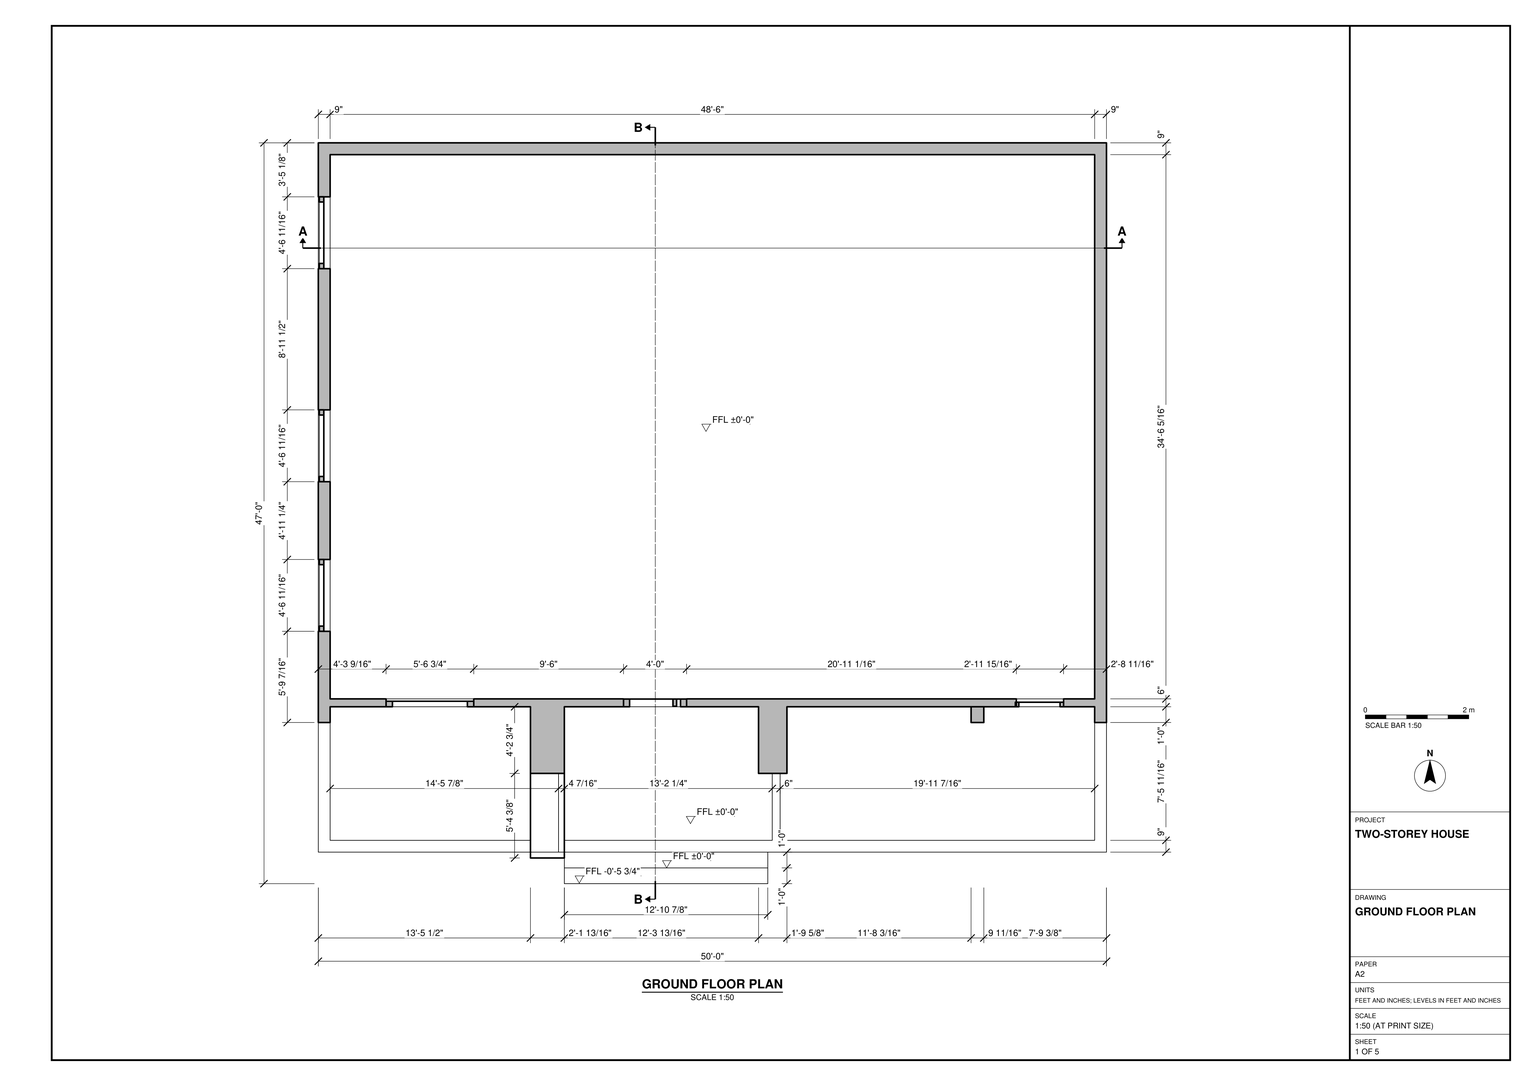
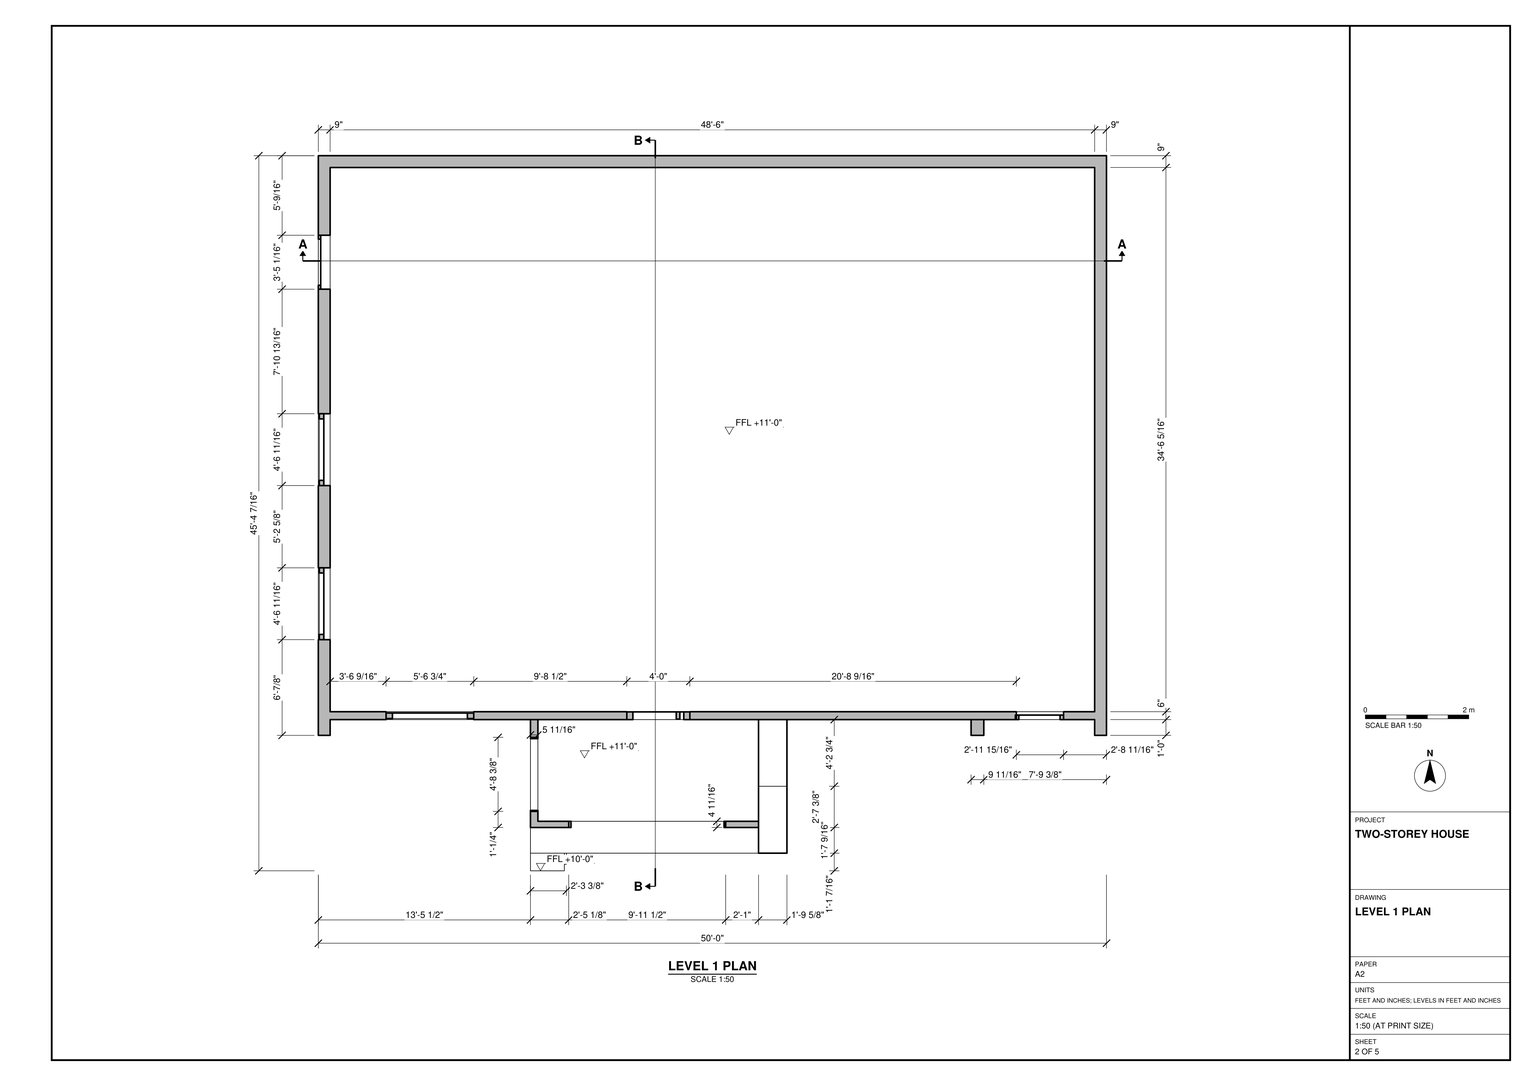
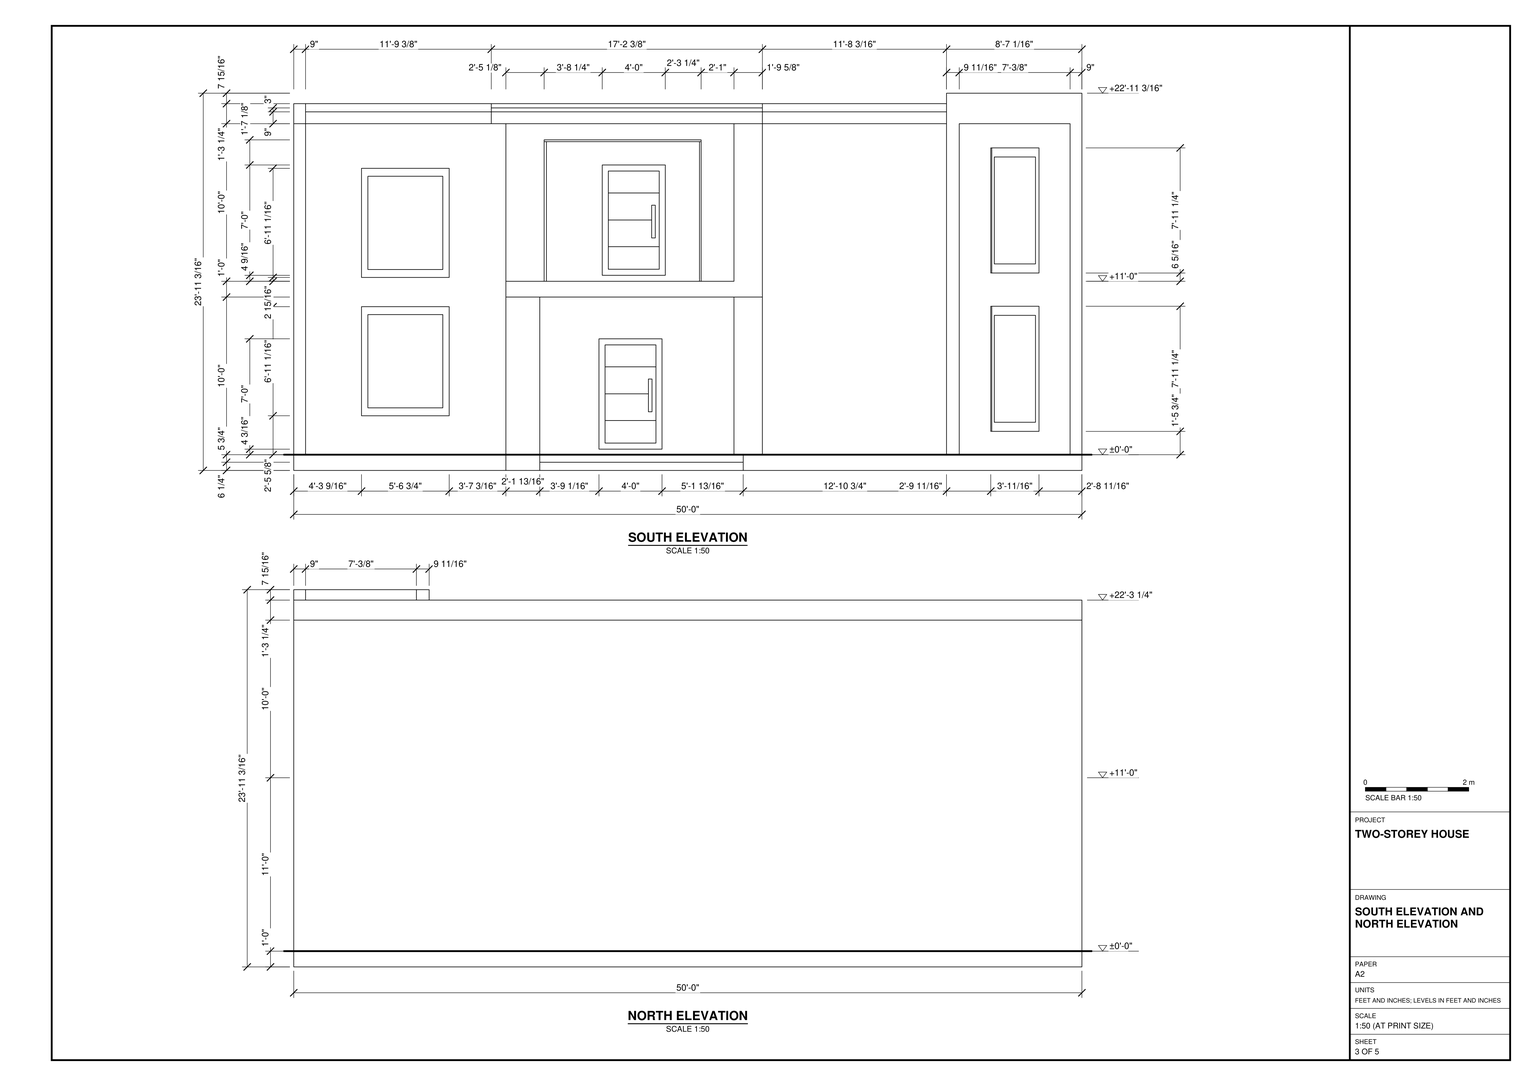
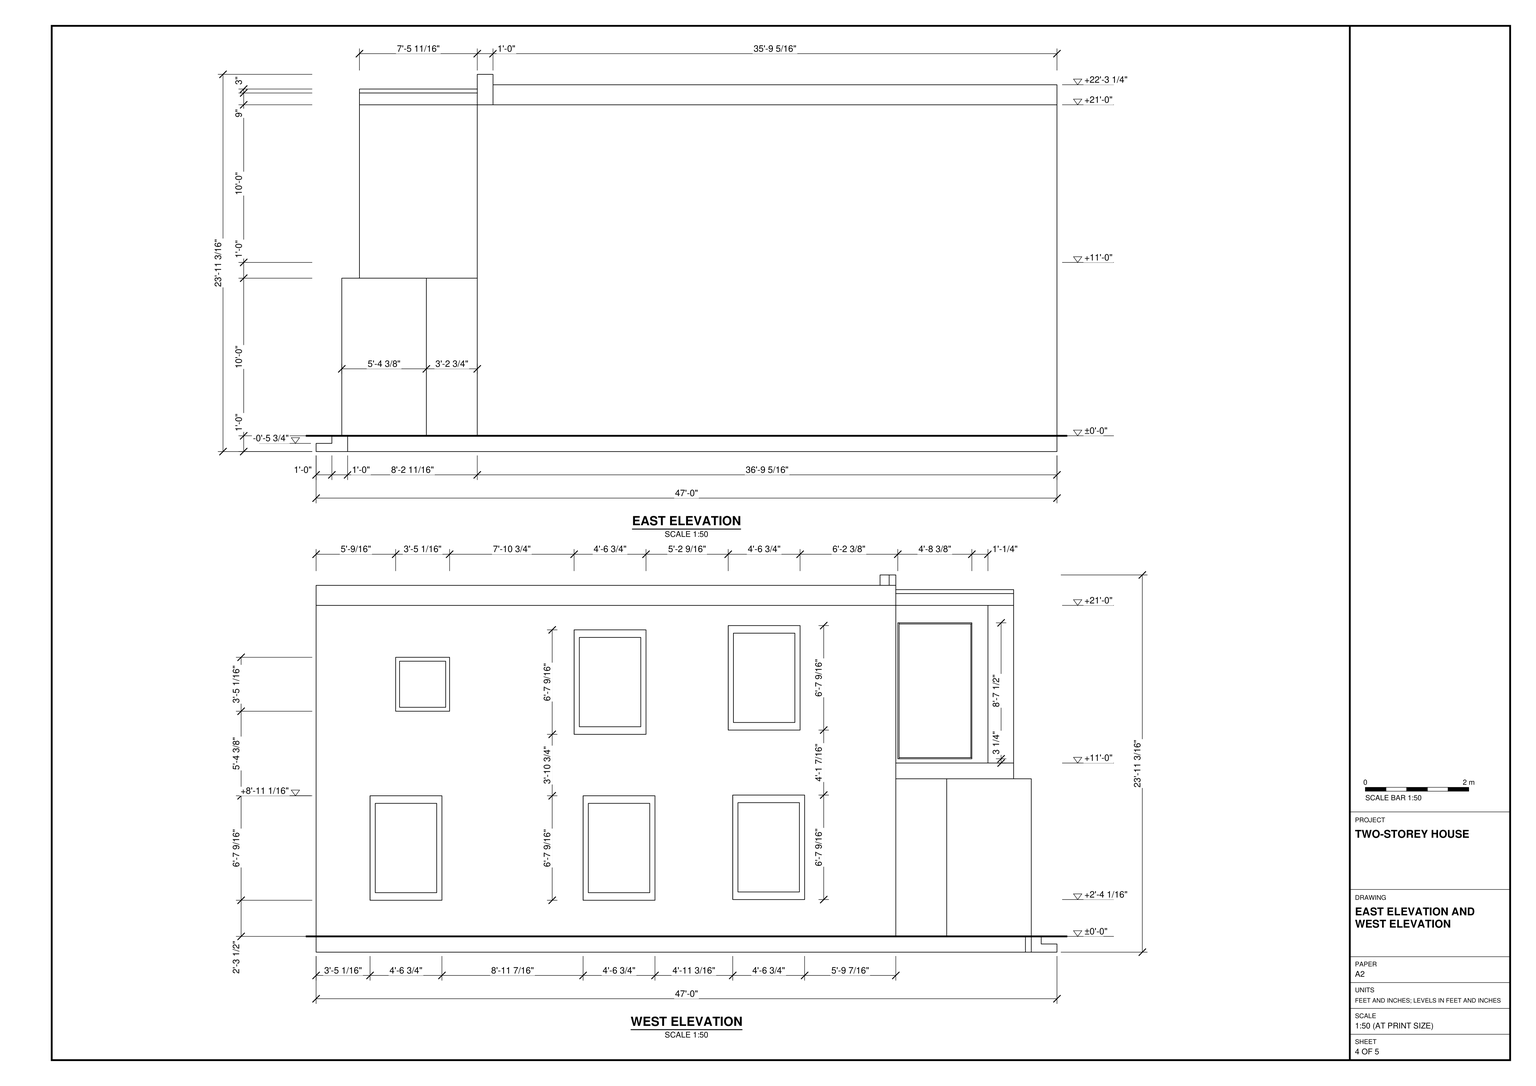
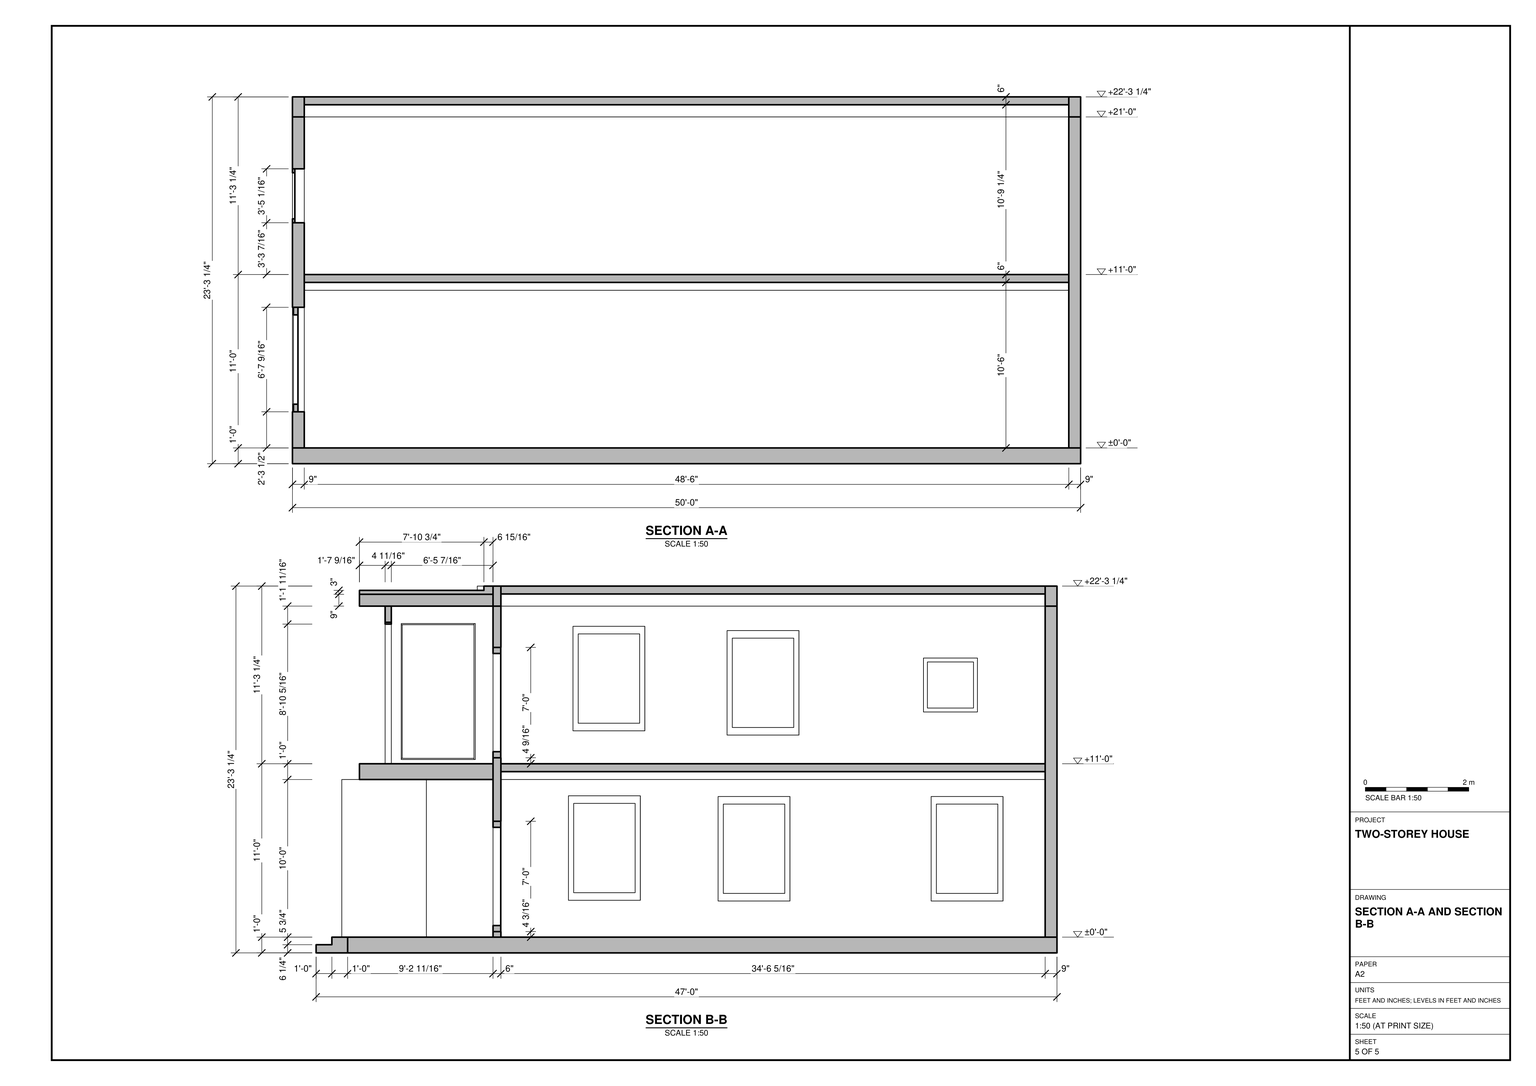
Build the two-storey house in SketchUp using task_files/diagram_01.pdf. Work in feet and inches. The overall model is 50'-0" wide, 47'-0" deep including the front steps, and 23'-11 3/16" high. Set the ground floor at ±0'-0" and the upper floor at +11'-0".

Use the plans to lay out the rectangular main shell, with 9" rear and side walls and a 6" front wall. Keep the floor areas open as drawn. Model the base, upper floor slab and flat roof, following the changes in roof-edge height on the south elevation. Build the steps up to the south porch and the projecting upper landing above it. Set the doors back from the front edge of the projection. Fit the wider front windows to the left of the entrance and the tall, narrow windows in the raised frame to the right. Use each floor plan for the spacing of the west windows rather than copying one storey onto the other.

Keep walls, slabs, roof and porch elements in separate groups or components. Keep each furniture or joinery piece separate where shown, and use components for repeated parts. Any decor or loose items shown may be represented by suitable library components. Save one SketchUp model as output_files/two_storey_house_with_a_projecting_entrance_porch.skp.

# SketchUp Ruby script. Lengths in inches.
U = 1.inch
M = Sketchup.active_model
def pt(a) = Geom::Point3d.new(a.map { |v| v * U })
def face(e, loops, mat)
  f = e.add_face(loops[0].map { |a| pt(a) })
  loops[1..].each { |l| e.add_face(l.map { |a| pt(a) }).erase! }
  f.material = f.back_material = mat if mat
  f
end
# faces: each face lists its corners as indices into pts; further lists are holes
def faces(e, pts, list, mat = nil) = list.each { |f| face(e, (f[0].is_a?(Array) ? f : [f]).map { |l| l.map { |i| pts[i] } }, mat) }
# xy, xz, yz: faces in a plane at the given z, y or x. An outline is a flat list of corners, or four numbers for a rectangle; further outlines are holes
def ring(l) = l.size == 4 ? [[l[0], l[1]], [l[2], l[1]], [l[2], l[3]], [l[0], l[3]]] : l.each_slice(2).to_a
def flat(e, list, mat, &to3) = list.each { |f| face(e, (f[0].is_a?(Array) ? f : [f]).map { |l| ring(l).map { |u, v| to3.(u, v) } }, mat) }
def xy(e, z, list, mat = nil) = flat(e, list, mat) { |x, y| [x, y, z] }
def xz(e, y, list, mat = nil) = flat(e, list, mat) { |x, z| [x, y, z] }
def yz(e, x, list, mat = nil) = flat(e, list, mat) { |y, z| [x, y, z] }
def lines(e, pts, list) = list.each { |a, b| e.add_line(pt(pts[a]), pt(pts[b])) }
# prism: a flat outline (further loops are holes) pulled along v
def prism(e, loops, v, mat = nil)
  f = face(e, loops, mat); d = Geom::Vector3d.new(v.map { |x| x * U })
  f.pushpull(f.normal.samedirection?(d) ? d.length : -d.length)
end
def box(e, o, s, mat = nil) = prism(e, [[o, [o[0] + s[0], o[1], o[2]], [o[0] + s[0], o[1] + s[1], o[2]], [o[0], o[1] + s[1], o[2]]]], [0, 0, s[2]], mat)
def at(x, y, z, deg = 0) = Geom::Transformation.translation(pt([x, y, z])) * Geom::Transformation.rotation(ORIGIN, Z_AXIS, deg.degrees)
def axes(o, x, y, z) = Geom::Transformation.new([*x, 0, *y, 0, *z, 0, *pt(o).to_a, 1])
def part(name) = M.definitions.add(name)
# library, detail: a bought-in or finely detailed component or shape, given as its bounding box
def library(name, o, s) = part(name).tap { |d| box(d.entities, o, s) }
def detail(e, o, s) = box(e.add_group.entities, o, s)
def put(e, d, t, mat = nil) = e.add_instance(d, t).tap { |i| i.material = mat if mat }
def group(e, t, mat = nil) = e.add_group.tap { |g| g.transformation = t; g.material = mat if mat }.entities
root = M.entities
M.materials.add("[Color D07]").color = [153, 134, 96]
M.materials.add("[Color M05]").color = [114, 114, 114]
M.materials.add("[Translucent Glass Gray]").color = [128, 128, 128]
M.materials["[Translucent Glass Gray]"].alpha = 0.5
c1 = part("Group\#1")
xy(c1.entities,0,[[0,0,48,5.875]],"[Color D07]")
xy(c1.entities,4.625,[[4.625,0,43.375,5.875]],"[Color D07]")
xy(c1.entities,28.45,[[37.63,0.375,40.38,5.875]],"[Color D07]")
xy(c1.entities,53.39,[[37.63,0.375,40.38,5.875]],"[Color D07]")
xy(c1.entities,79.375,[[4.625,0,43.375,5.875]],"[Color D07]")
xy(c1.entities,84,[[0,0,48,5.875]],"[Color D07]")
xz(c1.entities,0,[[[0,0,48,84],[4.625,4.625,43.375,79.375]]],"[Color D07]")
xz(c1.entities,0.375,[[37.63,28.45,40.38,53.39]],"[Color D07]")
xz(c1.entities,5.875,[[[0,0,48,84],[4.625,4.625,43.375,79.375]],[4.625,4.625,43.375,21.8],[4.625,21.8,43.375,21.8,43.375,62.68,4.625,62.68,4.625,42.12,37.63,42.12,37.63,53.39,40.38,53.39,40.38,28.45,37.63,28.45,37.63,42.12,4.625,42.12],[37.63,28.45,40.38,42.12],[37.63,42.12,40.38,53.39],
  [4.625,62.68,43.375,79.375]],"[Color D07]")
yz(c1.entities,0,[[0,0,5.875,84]],"[Color D07]")
yz(c1.entities,4.625,[[0,4.625,5.875,79.375]],"[Color D07]")
yz(c1.entities,37.63,[[0.375,28.45,5.875,53.39]],"[Color D07]")
yz(c1.entities,40.38,[[0.375,28.45,5.875,53.39]],"[Color D07]")
yz(c1.entities,43.375,[[0,4.625,5.875,79.375]],"[Color D07]")
yz(c1.entities,48,[[0,0,5.875,84]],"[Color D07]")
c2 = part("Group\#2")
xy(c2.entities,0,[[0,0,70.4375,5]],"[Color D07]")
xy(c2.entities,5.12,[[5.12,0,65.32,5]],"[Color D07]")
xy(c2.entities,65.32,[[5.12,0,65.32,5]],"[Color D07]")
xy(c2.entities,70.4375,[[0,0,70.4375,5]],"[Color D07]")
xz(c2.entities,0,[[[0,0,70.4375,70.4375],[5.12,5.12,65.32,65.32]]],"[Color D07]")
xz(c2.entities,5,[[[0,0,70.4375,70.4375],[5.12,5.12,65.32,65.32]]],"[Color D07]")
xz(c2.entities,5,[[5.12,5.12,65.32,65.32]],"[Translucent Glass Gray]")
yz(c2.entities,0,[[0,0,5,70.4375]],"[Color D07]")
yz(c2.entities,5.12,[[0,5.12,5,65.32]],"[Color D07]")
yz(c2.entities,65.32,[[0,5.12,5,65.32]],"[Color D07]")
yz(c2.entities,70.4375,[[0,0,5,70.4375]],"[Color D07]")
xy(root,0,[[187.29,0,342.17,24],[161.5,19.5625,187.29,24],[0,24,600,564]])
xy(root,6.24,[[187.29,0,342.17,12]],"[Color M05]")
xy(root,12,[[161.5,24,182.875,83.9375],[182.875,24,187.29,83.9375],[9,33,161.5,134.6875],[351.5625,33,591,33,591,134.6875,506.62,134.6875,506.62,122.6875,496.93,122.6875,496.93,134.6875,356.75,134.6875,356.75,83.9375,351.5625,83.9375],[[161.5,83.9375,161.5,134.6875,9,134.6875,9,122.6875,0,122.6875,0,564,600,564,600,122.6875,591,122.6875,591,134.6875,356.75,134.6875,356.75,83.9375,335.125,83.9375,335.125,134.6875,187.29,134.6875,187.29,83.9375],[9,140.6875,591,555]],
  [496.93,122.6875,506.62,134.6875],[9,140.6875,591,555]])
xy(root,12,[[187.29,12,342.17,24],[0,24,161.5,24,161.5,33,9,33,9,122.6875,0,122.6875],[187.29,24,600,24,600,122.6875,591,122.6875,591,33,351.5625,33,351.5625,83.9375,345.5625,83.9375,345.5625,33,187.29,33],[187.29,33,345.5625,33,345.5625,83.9375,335.125,83.9375,335.125,134.6875,187.29,134.6875]],"[Color M05]")
xy(root,16.21,[[232.36,134.6875,280.36,140.6875]])
xy(root,29.75,[[531.39,134.6875,567.33,140.6875]])
xy(root,39.51,[[0,306.02,9,360.71],[0,468.21,9,522.89]])
xy(root,40.04,[[0,192.11,9,246.8]])
xy(root,41.625,[[51.58,134.6875,118.33,140.6875]])
xy(root,100.21,[[232.36,134.6875,280.36,140.6875]])
xy(root,119.07,[[0,306.02,9,360.71],[0,468.21,9,522.89]])
xy(root,119.61,[[0,192.11,9,246.8]])
xy(root,124.6875,[[51.58,134.6875,118.33,140.6875]])
xy(root,125,[[531.39,134.6875,567.33,140.6875]])
xy(root,132,[[187.29,24.5625,188.875,33],[161.5,33,187.29,83.9375],[187.29,33,188.875,83.9375],[335.125,33,356.75,83.9375],[161.5,83.9375,187.29,134.6875],
  [335.125,83.9375,356.75,134.6875]])
xy(root,132,[[161.5,19.5625,187.29,33],[188.875,33,188.875,83.9375,187.29,83.9375,187.29,134.6875,335.125,134.6875,335.125,33]],"[Color M05]")
xy(root,138,[[9,140.6875,591,555]])
xy(root,144,[[161.5,52.54,161.5,134.6875,167.17,134.6875,167.17,57.26,190.62,57.26,190.62,52.54],[190.62,52.54,192.37,57.26],[308.87,52.54,310.12,57.26],[310.12,52.54,335.125,57.26],[167.17,57.26,335.125,134.6875],
  [9,140.6875,591,555]])
xy(root,144,[[161.5,33,335.125,33,335.125,52.54,308.87,52.54,308.87,57.26,192.37,57.26,192.37,52.54,161.5,52.54]],"[Color M05]")
xy(root,146.9375,[[51.58,134.6875,118.33,140.6875]])
xy(root,147.23,[[161.5,64.8125,167.17,120.1875],[161.5,120.1875,167.17,121.1875]])
xy(root,148.11,[[161.5,64.8125,167.17,65.5625],[161.5,65.5625,167.17,120.1875]])
xy(root,148.56,[[234.85,134.6875,282.85,140.6875]])
xy(root,150.3125,[[531.39,134.6875,567.33,140.6875]])
xy(root,165.83,[[0,312.86,9,367.54]])
xy(root,169.07,[[0,195.55,9,250.24]])
xy(root,183.42,[[0,462.37,9,503.43]])
xy(root,224.48,[[0,462.37,9,503.43]])
xy(root,230,[[51.58,134.6875,118.33,140.6875]])
xy(root,232.56,[[234.85,134.6875,282.85,140.6875]])
xy(root,245.39,[[0,312.86,9,367.54]])
xy(root,245.5625,[[531.39,134.6875,567.33,140.6875]])
xy(root,248.63,[[0,195.55,9,250.24]])
xy(root,249.86,[[161.5,64.8125,167.17,65.5625],[161.5,65.5625,167.17,120.1875]])
xy(root,250.32,[[190.62,52.54,192.37,57.26],[192.37,52.54,308.87,57.26],[308.87,52.54,310.12,57.26]])
xy(root,250.73,[[161.5,64.8125,167.17,120.1875],[161.5,120.1875,167.17,121.1875]])
xy(root,251.69,[[190.62,52.54,310.12,57.26]])
xy(root,264,[[335.125,33,356.75,134.6875],[161.5,52.54,167.17,134.6875],[167.17,52.54,335.125,57.26],[167.17,57.26,335.125,134.6875],[[0,122.6875,0,564,600,564,600,134.6875,9,134.6875,9,122.6875],[9,140.6875,591,555]]])
xy(root,264,[[150.375,33,150.375,134.6875,161.5,134.6875,161.5,52.54,335.125,52.54,335.125,33],[506.62,122.6875,591,134.6875]],"[Color M05]")
xy(root,273,[[150.375,33,356.75,134.6875],[9,127.75,150.375,134.6875],[356.75,127.75,496.93,134.6875]])
xy(root,273.25,[[9,140.6875,591,555]])
xy(root,276,[[150.375,33,356.75,127.75]],"[Color M05]")
xy(root,279.25,[[9,140.6875,591,555]])
xy(root,279.25,[[[0,122.6875,9,122.6875,9,134.6875,600,134.6875,600,564,0,564],[9,140.6875,591,555]],[9,127.75,496.93,134.6875]],"[Color M05]")
xy(root,287.1875,[[496.93,122.6875,600,134.6875]],"[Color M05]")
xz(root,0,[[187.29,0,342.17,6.24]],"[Color M05]")
xz(root,12,[[187.29,6.24,342.17,12]],"[Color M05]")
xz(root,19.5625,[[161.5,0,187.29,132]],"[Color M05]")
xz(root,24,[[0,0,161.5,12],[161.5,0,182.875,12],[182.875,0,187.29,12],[187.29,0,342.17,6.24],[342.17,0,600,12],
  [187.29,6.24,342.17,12]])
xz(root,33,[[161.5,132,356.75,132,356.75,264,335.125,264,335.125,144,161.5,144],[150.375,264,356.75,273],[150.375,273,356.75,276]],"[Color M05]")
xz(root,52.54,[[161.5,144,190.62,144,190.62,251.69,310.12,251.69,310.12,144,335.125,144,335.125,264,161.5,264],[190.62,144,192.37,250.32],[308.87,144,310.12,250.32],[190.62,250.32,310.12,251.69]])
xz(root,57.26,[[167.17,144,167.17,264,335.125,264,335.125,144,310.12,144,310.12,251.69,190.62,251.69,190.62,144],[190.62,144,192.37,250.32],[308.87,144,310.12,250.32],[190.62,250.32,310.12,251.69]])
xz(root,64.8125,[[161.5,147.23,167.17,148.11],[161.5,148.11,167.17,249.86],[161.5,249.86,167.17,250.73]])
xz(root,65.5625,[[161.5,148.11,167.17,249.86]])
xz(root,83.9375,[[161.5,12,187.29,132],[335.125,12,356.75,132]])
xz(root,120.1875,[[161.5,147.23,167.17,148.11],[161.5,148.11,167.17,249.86],[161.5,249.86,167.17,250.73]])
xz(root,121.1875,[[161.5,147.23,167.17,250.73]])
xz(root,122.6875,[[0,12,9,264],[0,264,9,279.25]])
xz(root,122.6875,[[496.93,12,506.62,12,506.62,264,591,264,591,12,600,12,600,287.1875,496.93,287.1875]],"[Color M05]")
xz(root,127.75,[[9,273,150.375,279.25],[356.75,273,496.93,279.25],[150.375,276,356.75,279.25]],"[Color M05]")
xz(root,134.6875,[[[9,12,161.5,264],[51.58,146.9375,118.33,230],[51.58,41.625,118.33,124.6875]],[[187.29,12,335.125,132],[232.36,16.21,280.36,100.21]],[356.75,12,496.93,264],[496.93,12,506.62,264],[[506.62,12,591,264],[531.39,150.3125,567.33,245.5625],[531.39,29.75,567.33,125]],
  [161.5,132,161.5,144,335.125,144,335.125,264,356.75,264,356.75,132],[161.5,144,167.17,264],[[167.17,144,335.125,264],[234.85,148.56,282.85,232.56]],[9,264,150.375,273],[150.375,264,176.17,273],
  [176.17,264,356.75,273],[356.75,264,496.93,273],[496.93,264,506.62,279.25],[506.62,264,591,279.25],[591,264,600,279.25],
  [9,273,161.5,279.25],[161.5,273,167.17,279.25],[167.17,273,176.17,279.25],[176.17,273,335.125,279.25],[335.125,273,496.93,279.25],
  [496.93,279.25,506.62,287.1875],[506.62,279.25,591,287.1875],[591,279.25,600,287.1875]])
xz(root,140.6875,[[[9,12,591,132],[51.58,41.625,118.33,124.6875],[232.36,16.21,280.36,100.21],[531.39,29.75,567.33,125]],[9,132,591,138],[9,138,591,144],[[9,144,591,264],[51.58,146.9375,118.33,230],[234.85,148.56,282.85,232.56],[531.39,150.3125,567.33,245.5625]],[9,264,591,273.25],
  [9,273.25,591,279.25]])
xz(root,192.11,[[0,40.04,9,119.61]])
xz(root,195.55,[[0,169.07,9,248.63]])
xz(root,246.8,[[0,40.04,9,119.61]])
xz(root,250.24,[[0,169.07,9,248.63]])
xz(root,306.02,[[0,39.51,9,119.07]])
xz(root,312.86,[[0,165.83,9,245.39]])
xz(root,360.71,[[0,39.51,9,119.07]])
xz(root,367.54,[[0,165.83,9,245.39]])
xz(root,462.37,[[0,183.42,9,224.48]])
xz(root,468.21,[[0,39.51,9,119.07]])
xz(root,503.43,[[0,183.42,9,224.48]])
xz(root,522.89,[[0,39.51,9,119.07]])
xz(root,555,[[9,12,591,132],[9,132,591,138],[9,138,591,144],[9,144,591,264],[9,264,591,273.25],
  [9,273.25,32.25,279.25],[32.25,273.25,591,279.25]])
xz(root,564,[[0,0,600,12],[0,12,600,264],[0,264,600,279.25]])
yz(root,0,[[24,0,564,12],[[122.6875,12,564,264],[192.11,40.04,246.8,119.61],[306.02,39.51,360.71,119.07],[468.21,39.51,522.89,119.07],[195.55,169.07,250.24,248.63],[312.86,165.83,367.54,245.39],[462.37,183.42,503.43,224.48]],[122.6875,264,564,279.25]])
yz(root,9,[[122.6875,12,134.6875,132],[[140.6875,12,555,132],[468.21,39.51,522.89,119.07],[306.02,39.51,360.71,119.07],[192.11,40.04,246.8,119.61]],[122.6875,132,134.6875,144],[140.6875,132,555,138],[140.6875,138,183.61,144],
  [183.61,138,208.99,144],[208.99,138,555,144],[122.6875,144,134.6875,264],[[140.6875,144,555,264],[312.86,165.83,367.54,245.39],[195.55,169.07,250.24,248.63],[462.37,183.42,503.43,224.48]],[122.6875,264,134.6875,264,134.6875,273,127.75,273,127.75,279.25,122.6875,279.25],
  [140.6875,264,555,273.25],[140.6875,273.25,555,279.25]])
yz(root,51.58,[[134.6875,41.625,140.6875,124.6875],[134.6875,146.9375,140.6875,230]])
yz(root,118.33,[[134.6875,41.625,140.6875,124.6875],[134.6875,146.9375,140.6875,230]])
yz(root,150.375,[[33,264,134.6875,273],[33,273,127.75,276]],"[Color M05]")
yz(root,161.5,[[83.9375,12,134.6875,132],[[52.54,144,134.6875,264],[64.8125,147.23,121.1875,250.73]],[64.8125,147.23,120.1875,148.11],[120.1875,147.23,121.1875,250.73],[64.8125,148.11,65.5625,249.86],
  [64.8125,249.86,120.1875,250.73]])
yz(root,161.5,[[19.5625,0,19.5625,132,83.9375,132,83.9375,12,24,12,24,0],[33,132,134.6875,144]],"[Color M05]")
yz(root,167.17,[[[57.26,144,134.6875,264],[64.8125,147.23,121.1875,250.73]],[64.8125,147.23,120.1875,148.11],[120.1875,147.23,121.1875,250.73],[64.8125,148.11,65.5625,249.86],[64.8125,249.86,120.1875,250.73]])
yz(root,187.29,[[19.5625,0,24,12],[83.9375,12,134.6875,132]])
yz(root,187.29,[[0,0,0,6.24,12,6.24,12,12,19.5625,12,19.5625,0],[19.5625,12,83.9375,132]],"[Color M05]")
yz(root,190.62,[[52.54,144,57.26,250.32],[52.54,250.32,57.26,251.69]])
yz(root,192.37,[[52.54,144,57.26,250.32]])
yz(root,232.36,[[134.6875,16.21,140.6875,100.21]])
yz(root,234.85,[[134.6875,148.56,140.6875,232.56]])
yz(root,280.36,[[134.6875,16.21,140.6875,100.21]])
yz(root,282.85,[[134.6875,148.56,140.6875,232.56]])
yz(root,308.87,[[52.54,144,57.26,250.32]])
yz(root,310.12,[[52.54,144,57.26,250.32],[52.54,250.32,57.26,251.69]])
yz(root,335.125,[[83.9375,12,134.6875,132],[52.54,144,57.26,264],[57.26,144,134.6875,264]])
yz(root,335.125,[[33,144,52.54,264]],"[Color M05]")
yz(root,342.17,[[0,0,24,0,24,12,12,12,12,6.24,0,6.24]],"[Color M05]")
yz(root,356.75,[[83.9375,12,134.6875,132]])
yz(root,356.75,[[33,132,134.6875,264],[33,264,127.75,273],[127.75,264,134.6875,273],[33,273,127.75,276]],"[Color M05]")
yz(root,496.93,[[122.6875,12,122.6875,287.1875,127.75,287.1875,127.75,273,134.6875,273,134.6875,12],[127.75,279.25,134.6875,287.1875]],"[Color M05]")
yz(root,506.62,[[122.6875,12,134.6875,264]],"[Color M05]")
yz(root,531.39,[[134.6875,29.75,140.6875,125],[134.6875,150.3125,140.6875,245.5625]])
yz(root,567.33,[[134.6875,29.75,140.6875,125],[134.6875,150.3125,140.6875,245.5625]])
yz(root,591,[[140.6875,12,555,132],[140.6875,132,555,138],[140.6875,138,555,144],[140.6875,144,555,264],[140.6875,264,555,273.25],
  [140.6875,273.25,555,279.25]])
yz(root,591,[[122.6875,12,134.6875,132],[122.6875,132,134.6875,144],[122.6875,144,134.6875,264]],"[Color M05]")
yz(root,600,[[24,0,564,12],[122.6875,12,564,264],[134.6875,264,564,279.25]])
yz(root,600,[[122.6875,264,134.6875,287.1875]],"[Color M05]")
put(root,c1,at(234.85,134.6875,148.56))
put(root,c1,at(232.36,134.6875,16.21))
put(root,c2,axes([51.58,135.49,146.9375],[0.94765,0,0],[0,0.84,0],[0,0,1.17924]))
put(root,c2,axes([51.58,134.6875,41.625],[0.94765,0,0],[0,0.84,0],[0,0,1.17924]))
put(root,c2,axes([530.62,134.6875,150.3125],[0.52121,0,0],[0,0.6888,0],[0,0,1.35226]))
put(root,c2,axes([530.62,134.6875,29.75],[0.52121,0,0],[0,0.6888,0],[0,0,1.35226]))
put(root,c2,axes([0.76,250.29,169.07],[0,-0.77707,0],[0.6888,0,0],[0,0,1.12955]))
put(root,c2,axes([0.76,246.84,40.04],[0,-0.77707,0],[0.6888,0,0],[0,0,1.12955]))
put(root,c2,axes([0.76,360.75,39.51],[0,-0.77707,0],[0.6888,0,0],[0,0,1.12955]))
put(root,c2,axes([0.76,367.59,165.83],[0,-0.77707,0],[0.6888,0,0],[0,0,1.12955]))
put(root,c2,axes([0.76,522.94,39.51],[0,-0.77707,0],[0.6888,0,0],[0,0,1.12955]))
put(root,c2,axes([0,503.43,183.42],[0,-0.58296,0],[0.36531,0,0],[0,0,0.58296]))
